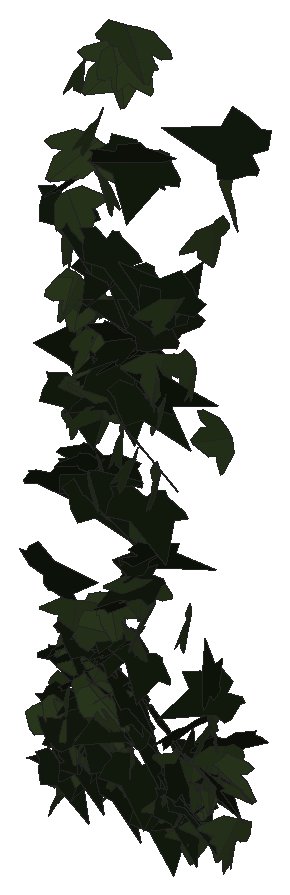
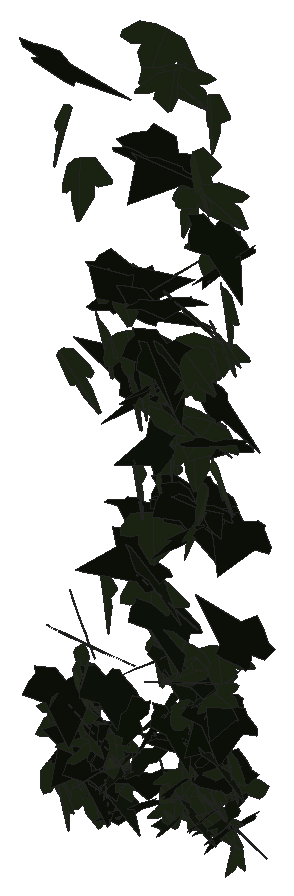
# SketchUp Ruby script. Lengths in inches.
U = 1.inch
M = Sketchup.active_model
def pt(a) = Geom::Point3d.new(a.map { |v| v * U })
def face(e, loops, mat)
  f = e.add_face(loops[0].map { |a| pt(a) })
  loops[1..].each { |l| e.add_face(l.map { |a| pt(a) }).erase! }
  f.material = f.back_material = mat if mat
  f
end
# faces: each face lists its corners as indices into pts; further lists are holes
def faces(e, pts, list, mat = nil) = list.each { |f| face(e, (f[0].is_a?(Array) ? f : [f]).map { |l| l.map { |i| pts[i] } }, mat) }
# xy, xz, yz: faces in a plane at the given z, y or x. An outline is a flat list of corners, or four numbers for a rectangle; further outlines are holes
def ring(l) = l.size == 4 ? [[l[0], l[1]], [l[2], l[1]], [l[2], l[3]], [l[0], l[3]]] : l.each_slice(2).to_a
def flat(e, list, mat, &to3) = list.each { |f| face(e, (f[0].is_a?(Array) ? f : [f]).map { |l| ring(l).map { |u, v| to3.(u, v) } }, mat) }
def xy(e, z, list, mat = nil) = flat(e, list, mat) { |x, y| [x, y, z] }
def xz(e, y, list, mat = nil) = flat(e, list, mat) { |x, z| [x, y, z] }
def yz(e, x, list, mat = nil) = flat(e, list, mat) { |y, z| [x, y, z] }
def lines(e, pts, list) = list.each { |a, b| e.add_line(pt(pts[a]), pt(pts[b])) }
# prism: a flat outline (further loops are holes) pulled along v
def prism(e, loops, v, mat = nil)
  f = face(e, loops, mat); d = Geom::Vector3d.new(v.map { |x| x * U })
  f.pushpull(f.normal.samedirection?(d) ? d.length : -d.length)
end
def box(e, o, s, mat = nil) = prism(e, [[o, [o[0] + s[0], o[1], o[2]], [o[0] + s[0], o[1] + s[1], o[2]], [o[0], o[1] + s[1], o[2]]]], [0, 0, s[2]], mat)
def at(x, y, z, deg = 0) = Geom::Transformation.translation(pt([x, y, z])) * Geom::Transformation.rotation(ORIGIN, Z_AXIS, deg.degrees)
def axes(o, x, y, z) = Geom::Transformation.new([*x, 0, *y, 0, *z, 0, *pt(o).to_a, 1])
def part(name) = M.definitions.add(name)
# library, detail: a bought-in or finely detailed component or shape, given as its bounding box
def library(name, o, s) = part(name).tap { |d| box(d.entities, o, s) }
def detail(e, o, s) = box(e.add_group.entities, o, s)
def put(e, d, t, mat = nil) = e.add_instance(d, t).tap { |i| i.material = mat if mat }
def group(e, t, mat = nil) = e.add_group.tap { |g| g.transformation = t; g.material = mat if mat }.entities
root = M.entities
M.materials.add("1026 AP 7946 SUNNY SIDE UP").color = [254, 231, 186]
M.materials.add("efeu1").color = [18, 25, 13]
M.materials.add("efeu2").color = [43, 57, 29]
c1 = part("ivyleaf_10")
p = [[0,0.5,-0.03],[-0.0625,2.02,-0.43],[-0.19,2.01,-0.46],[-0.54,1.05,-0.29],[-0.52,0.625,-0.18],[-0.83,0.76,-0.28],
  [-1.16,0.64,-0.33],[-1.15,0.33,-0.24],[-0.77,-0.39,0.02],[-0.3,-0.51,0.16],[0.04,-0.48,0.23],[-0.02,2.01,-0.4375],
  [-0.06,2.01,-0.43],[0.04,-0.49,0.23],[0.67,-0.49,0.14],[1.38,0.36,-0.2],[1.375,0.51,-0.24],[0.81,0.65,-0.19],
  [0.62,0.59,-0.15],[0.6,1.09,-0.28],[0.5,1.23,-0.31]]
faces(c1.entities,p,[[0,1,2,3,4,5,6,7,8,9,10],[11,12,0,13,14,15,16,17,18,19,20]],"efeu2")
c2 = part("ivyleaf_9")
p = [[1.54,2.16,1.25],[1.36,2.04,1.19],[-0.21,0.99,0.68],[-0.71,1.11,0.82],[-0.85,0.86,0.67],[-0.8,0.17,0.21],
  [-0.9,-0.01,0.1],[-0.67,-0.16,-0.02],[-0.08,-0.08,-0.05],[-0.03,-0.6,-0.4],[0.65,-0.88,-0.66],[0.83,-0.6,-0.49],
  [1.29,-0.42,-0.43],[1.8125,-0.07,-0.26],[1.21,0.44,0.15]]
faces(c2.entities,p,[[0,1,2,3,4,5,6,7,8,9,10,11,12,13,14]],"efeu1")
put(root,c1,axes([99.48,212.96,273.32],[-0.02906,0.13173,0.21889],[-0.30626,0.12835,-0.1038],[-0.27324,-0.15787,0.09306]),"1026 AP 7946 SUNNY SIDE UP")
put(root,c1,axes([99.28,212.93,269.21],[0.26104,-0.20482,-0.03217],[0.01718,0.04715,-0.26851],[0.32505,0.16199,0.04003]),"1026 AP 7946 SUNNY SIDE UP")
put(root,c1,axes([99.33,212.97,275.96],[0.25724,-0.22713,-0.0943],[-0.00591,0.10625,-0.28187],[0.38425,0.15368,0.05879]),"1026 AP 7946 SUNNY SIDE UP")
put(root,c2,axes([99.04,212.875,270.85],[0.02843,-0.03643,0.27976],[0.29208,-0.19871,-0.04134],[0.31714,0.18627,0.01299]),"1026 AP 7946 SUNNY SIDE UP")
put(root,c2,axes([99.59,212.82,268.3],[-0.23447,0.14999,0.07578],[-0.104,0.03674,-0.21682],[-0.26012,-0.14989,0.01838]),"1026 AP 7946 SUNNY SIDE UP")
put(root,c2,axes([99.51,212.96,276.91],[-0.07158,0.29227,-0.0364],[0.00245,-0.03719,-0.30491],[-0.46322,-0.04536,0.00402]),"1026 AP 7946 SUNNY SIDE UP")
put(root,c1,axes([99.38,212.6875,267.79],[-0.00639,-0.10073,-0.20656],[0.01108,0.19151,-0.10524],[0.36733,-0.00753,-0.00042]),"1026 AP 7946 SUNNY SIDE UP")
put(root,c2,axes([99.32,212.67,272.54],[0.26615,0.18266,-0.01135],[0.00617,-0.02019,-0.25743],[-0.3108,0.15602,-0.01483]),"1026 AP 7946 SUNNY SIDE UP")
put(root,c1,axes([99.16,212.77,268.875],[0.2529,0.11365,0.14396],[0.19708,0.06644,-0.19909],[-0.22215,0.18833,-0.01273]),"1026 AP 7946 SUNNY SIDE UP")
put(root,c1,axes([99.27,212.875,269.01],[0.14805,0.1932,0.05915],[0.04785,0.0451,-0.22619],[-0.33658,0.09139,-0.00614]),"1026 AP 7946 SUNNY SIDE UP")
put(root,c1,axes([99.42,213.03,270.15],[0.13651,0.14455,-0.1499],[-0.10188,-0.12882,-0.17869],[-0.32841,0.10005,-0.00687]),"1026 AP 7946 SUNNY SIDE UP")
put(root,c2,axes([99.72,212.87,274.45],[-0.04379,-0.02297,-0.29501],[-0.44997,-0.02165,0.03035],[-0.03748,0.28677,-0.01964]),"1026 AP 7946 SUNNY SIDE UP")
put(root,c2,axes([99.23,212.9,268.5],[0.24861,-0.20292,-0.05814],[-0.03895,0.05072,-0.26445],[0.3284,0.15963,0.01265]),"1026 AP 7946 SUNNY SIDE UP")
put(root,c2,axes([99.62,212.87,269.22],[-0.11625,0.20118,0.06581],[-0.06571,0.0487,-0.2258],[-0.3497,-0.07603,0.02055]),"1026 AP 7946 SUNNY SIDE UP")
put(root,c2,axes([99.44,212.87,269.83],[0.24397,0.14977,-0.08389],[-0.06946,-0.0716,-0.22232],[-0.28,0.14826,-0.01795]),"1026 AP 7946 SUNNY SIDE UP")
put(root,c2,axes([99.3,212.84,268.1875],[0.08772,-0.24399,-0.0776],[-0.01717,0.07334,-0.25735],[0.40052,0.05658,0.00596]),"1026 AP 7946 SUNNY SIDE UP")
put(root,c2,axes([99.48,212.79,270.02],[0.10433,0.20292,0.08704],[0.05126,0.07299,-0.22584],[-0.36587,0.06809,-0.00682]),"1026 AP 7946 SUNNY SIDE UP")
put(root,c1,axes([99.47,212.91,275.3],[0.29987,-0.17743,0.03416],[0.0212,-0.03575,-0.26798],[0.30601,0.17634,-0.01491]),"1026 AP 7946 SUNNY SIDE UP")
put(root,c2,axes([99.33,212.95,276.48],[0.05518,-0.29071,-0.04839],[-0.0112,0.04479,-0.3014],[0.46251,0.03577,-0.00152]),"1026 AP 7946 SUNNY SIDE UP")
put(root,c1,axes([99.58,212.82,270.58],[-0.27514,-0.15876,0.01353],[-0.00008,-0.02093,-0.24267],[0.27066,-0.1614,0.01368]),"1026 AP 7946 SUNNY SIDE UP")
put(root,c1,axes([99.64,212.89,268.63],[0.18742,-0.13295,-0.14177],[-0.13748,0.10261,-0.18356],[0.28505,0.1369,0.00468]),"1026 AP 7946 SUNNY SIDE UP")
put(root,c1,axes([99.63,212.93,268.2],[0.30089,0.03433,-0.12362],[-0.18268,-0.04895,-0.19237],[-0.09353,0.20606,-0.02198]),"1026 AP 7946 SUNNY SIDE UP")
put(root,c2,axes([99.29,212.95,268.93],[-0.01066,-0.02643,0.23627],[0.37545,-0.02589,0.00305],[0.04298,0.21961,0.03195]),"1026 AP 7946 SUNNY SIDE UP")
put(root,c1,axes([99.68,212.95,277.375],[0.37547,0.07924,-0.1682],[-0.22868,-0.07909,-0.25841],[-0.17176,0.27851,-0.02364]),"1026 AP 7946 SUNNY SIDE UP")
put(root,c1,axes([99.55,212.87,268.75],[0.11961,0.20132,-0.04717],[-0.02057,-0.04521,-0.22895],[-0.35022,0.07141,-0.00266]),"1026 AP 7946 SUNNY SIDE UP")
put(root,c1,axes([99.63,212.86,278.625],[0.04202,-0.24833,-0.11165],[0.01989,0.10238,-0.26486],[0.45467,0.01847,0.0219]),"1026 AP 7946 SUNNY SIDE UP")
put(root,c1,axes([99.54,212.95,275.21],[0.41653,0.05757,-0.00079],[0.00664,-0.02316,-0.26898],[-0.09753,0.24428,-0.02169]),"1026 AP 7946 SUNNY SIDE UP")
put(root,c1,axes([99.6,212.73,276.64],[0.13605,0.27126,0.08601],[-0.0259,0.09035,-0.28967],[-0.44482,0.0777,0.04317]),"1026 AP 7946 SUNNY SIDE UP")
put(root,c2,axes([99.6,212.8,269.52],[0.15571,0.15469,0.14055],[0.10084,0.11497,-0.19082],[-0.32701,0.10911,0.00808]),"1026 AP 7946 SUNNY SIDE UP")
put(root,c1,axes([99.71,213.16,274.98],[-0.06034,-0.2179,0.12437],[-0.01126,-0.11935,-0.23773],[0.42132,-0.0344,0.01146]),"1026 AP 7946 SUNNY SIDE UP")
put(root,c2,axes([99.64,212.72,268.61],[-0.29105,-0.01711,0.1575],[0.24634,0.02724,0.18456],[-0.05209,0.22442,-0.0072]),"1026 AP 7946 SUNNY SIDE UP")
put(root,c2,axes([99.54,212.95,273.78],[-0.14208,-0.21245,-0.09578],[0.11469,0.06538,-0.24043],[0.37225,-0.10123,0.03752]),"1026 AP 7946 SUNNY SIDE UP")
put(root,c2,axes([99.58,212.84,269.98],[0.20095,-0.1581,-0.11715],[-0.13095,0.07602,-0.20984],[0.29682,0.14058,-0.01326]),"1026 AP 7946 SUNNY SIDE UP")
put(root,c2,axes([99.54,212.93,268.38],[0.09931,-0.25091,-0.03775],[-0.0209,0.03296,-0.26631],[0.39785,0.06436,-0.00457]),"1026 AP 7946 SUNNY SIDE UP")
put(root,c1,axes([99.71,212.98,272.96],[-0.22119,0.20081,0.0047],[-0.02725,-0.00831,-0.25567],[-0.33981,-0.13005,0.01745]),"1026 AP 7946 SUNNY SIDE UP")
put(root,c2,axes([99.5,212.91,270.19],[0.21501,-0.21942,-0.0849],[-0.00202,0.09331,-0.26154],[0.36786,0.12876,0.04819]),"1026 AP 7946 SUNNY SIDE UP")
put(root,c1,axes([99.78,212.96,277.76],[0.06086,-0.29776,-0.03273],[-0.00454,0.02996,-0.30915],[0.47056,0.0388,0.00125]),"1026 AP 7946 SUNNY SIDE UP")
put(root,c1,axes([99.7,212.92,273.89],[-0.33973,-0.11641,-0.08991],[0.1576,0.0016,-0.2436],[0.18388,-0.21645,0.04266]),"1026 AP 7946 SUNNY SIDE UP")
put(root,c1,axes([99.78,212.91,268.77],[0.04086,-0.20317,0.08096],[0.02729,-0.07687,-0.22],[0.36859,0.02822,0.00732]),"1026 AP 7946 SUNNY SIDE UP")
put(root,c2,axes([99.82,213.0625,268.29],[-0.26926,0.02251,-0.14891],[0.19446,-0.10204,-0.15862],[-0.14011,-0.18487,0.06602]),"1026 AP 7946 SUNNY SIDE UP")
put(root,c1,axes([99.9,212.85,268.57],[-0.34195,-0.06555,0.06616],[-0.08761,-0.04262,-0.22597],[0.12657,-0.20661,0.02233]),"1026 AP 7946 SUNNY SIDE UP")
put(root,c1,axes([99.9,212.89,269.72],[-0.28529,-0.17399,0.09757],[-0.0401,-0.10814,-0.25299],[0.30965,-0.1743,0.05714]),"1026 AP 7946 SUNNY SIDE UP")
put(root,c1,axes([99.84,212.91,274.57],[0.17858,0.17914,-0.14354],[-0.12692,-0.11423,-0.22393],[-0.36054,0.12894,0.00774]),"1026 AP 7946 SUNNY SIDE UP")
put(root,c2,axes([99.93,212.87,272.83],[0.14729,0.21051,-0.17033],[-0.08716,-0.15741,-0.23803],[-0.41296,0.10831,-0.01051]),"1026 AP 7946 SUNNY SIDE UP")
put(root,c2,axes([99.99,212.87,272.92],[0.21407,0.1349,-0.21574],[-0.1958,-0.17084,-0.19705],[-0.34042,0.1831,-0.02233]),"1026 AP 7946 SUNNY SIDE UP")
put(root,c1,axes([99.84,212.89,272.5],[-0.11595,0.271,0.03562],[-0.01419,0.03178,-0.28915],[-0.42904,-0.07429,-0.00006]),"1026 AP 7946 SUNNY SIDE UP")
put(root,c1,axes([99.93,212.88,273.59],[-0.13026,-0.27077,-0.03588],[0.02259,0.03041,-0.29149],[0.42837,-0.08394,0.00446]),"1026 AP 7946 SUNNY SIDE UP")
put(root,c2,axes([99.91,213.12,275.68],[-0.3555,-0.03039,-0.15172],[0.24116,-0.08919,-0.2061],[-0.04528,-0.23638,0.09345]),"1026 AP 7946 SUNNY SIDE UP")
put(root,c1,axes([99.76,212.85,270.33],[-0.04557,-0.09391,-0.22584],[0.26716,0.14635,-0.08967],[0.28424,-0.15261,0.04808]),"1026 AP 7946 SUNNY SIDE UP")
put(root,c2,axes([99.67,212.9375,269.35],[0.32432,-0.07494,0.09486],[0.12733,-0.05292,-0.21939],[0.15197,0.20427,-0.01861]),"1026 AP 7946 SUNNY SIDE UP")
put(root,c1,axes([99.91,212.8,269.12],[-0.31655,0.0954,-0.0812],[0.10269,-0.0505,-0.22427],[-0.18113,-0.19536,0.01476]),"1026 AP 7946 SUNNY SIDE UP")
put(root,c2,axes([100.16,212.93,270.15],[-0.22318,0.1661,-0.06961],[0.02126,-0.07461,-0.22475],[-0.30341,-0.12741,0.03546]),"1026 AP 7946 SUNNY SIDE UP")
put(root,c2,axes([99.79,212.88,272.4],[0.12537,-0.21985,-0.16406],[0.01995,0.16756,-0.23262],[0.42524,0.05695,0.05928]),"1026 AP 7946 SUNNY SIDE UP")
put(root,c1,axes([100.07,212.77,277.13],[-0.29153,0.18982,0.05644],[-0.0697,0.03056,-0.27342],[-0.32596,-0.17631,0.00799]),"1026 AP 7946 SUNNY SIDE UP")
put(root,c1,axes([100,213.04,268.82],[0.15013,0.19121,-0.04039],[-0.02115,-0.03854,-0.22603],[-0.33102,0.08919,-0.00388]),"1026 AP 7946 SUNNY SIDE UP")
put(root,c2,axes([99.87,212.9,272.69],[-0.16585,-0.16563,-0.21064],[0.21774,0.15119,-0.1998],[0.35048,-0.17231,0.02445]),"1026 AP 7946 SUNNY SIDE UP")
put(root,c2,axes([99.99,213.18,270.21],[-0.21047,-0.18459,0.00949],[0.10301,-0.05343,-0.22284],[0.29656,-0.11245,0.08414]),"1026 AP 7946 SUNNY SIDE UP")
put(root,c2,axes([100.27,212.91,273.99],[-0.35524,0.11989,-0.03775],[-0.00129,-0.07284,-0.2503],[-0.2129,-0.19961,0.06451]),"1026 AP 7946 SUNNY SIDE UP")
put(root,c2,axes([100.18,212.97,269.51],[-0.01621,0.21772,0.01632],[-0.01153,0.01212,-0.23305],[-0.37002,-0.00991,0.00655]),"1026 AP 7946 SUNNY SIDE UP")
put(root,c1,axes([99.96,213.02,270.68],[0.35551,-0.00348,0.09238],[0.14556,-0.01948,-0.2238],[0.01806,0.22568,-0.01472]),"1026 AP 7946 SUNNY SIDE UP")
put(root,c1,axes([100.44,212.86,273.875],[0.03534,0.04698,0.29322],[-0.41166,-0.11595,0.04038],[0.18952,-0.26062,0.03302]),"1026 AP 7946 SUNNY SIDE UP")
put(root,c2,axes([100,212.9,268.65],[0.11642,-0.22462,-0.12154],[-0.04103,0.11417,-0.24277],[0.3959,0.07789,0.01058]),"1026 AP 7946 SUNNY SIDE UP")
put(root,c1,axes([99.98,212.76,269.43],[0.23136,0.12898,0.14159],[0.17872,0.07828,-0.19933],[-0.2552,0.17175,-0.01124]),"1026 AP 7946 SUNNY SIDE UP")
put(root,c1,axes([100.14,213.03,268.28],[0.14338,0.1858,-0.05314],[-0.02499,-0.05046,-0.21907],[-0.3266,0.08543,-0.00657]),"1026 AP 7946 SUNNY SIDE UP")
put(root,c1,axes([100.28,212.92,278.91],[0.40825,0.05973,-0.15606],[-0.21615,-0.07359,-0.27244],[-0.13817,0.29162,-0.0349]),"1026 AP 7946 SUNNY SIDE UP")
put(root,c2,axes([100.4,212.85,270.35],[-0.23754,0.18054,-0.10144],[0.00838,-0.11457,-0.23726],[-0.34789,-0.12603,0.06355]),"1026 AP 7946 SUNNY SIDE UP")
put(root,c2,axes([100.41,212.96,269.15],[-0.3875,-0.05497,0.05522],[-0.06866,-0.05214,-0.24838],[0.10897,-0.22831,0.03988]),"1026 AP 7946 SUNNY SIDE UP")
put(root,c2,axes([100.42,212.86,274.82],[-0.35603,0.13221,-0.10197],[0.08201,-0.10063,-0.26014],[-0.26597,-0.208,0.05629]),"1026 AP 7946 SUNNY SIDE UP")
put(root,c2,axes([100.04,212.92,276.12],[0.09562,-0.28949,-0.02436],[0.02882,0.02626,-0.30364],[0.4556,0.0591,0.02432]),"1026 AP 7946 SUNNY SIDE UP")
put(root,c1,axes([100.28,212.96,268.35],[0.02651,-0.18688,0.13091],[0.01109,-0.12459,-0.20247],[0.38123,0.01662,-0.00322]),"1026 AP 7946 SUNNY SIDE UP")
put(root,c2,axes([100.1,212.9375,268.13],[0.14393,-0.24195,0.01973],[0.00408,-0.02096,-0.26657],[0.38178,0.09144,-0.00459]),"1026 AP 7946 SUNNY SIDE UP")
put(root,c2,axes([100.37,212.88,274.87],[0.29758,0.11706,-0.17039],[-0.24601,-0.07141,-0.22595],[-0.23102,0.22683,0.02113]),"1026 AP 7946 SUNNY SIDE UP")
put(root,c1,axes([100.22,212.95,278.91],[0.17131,0.28486,-0.03155],[-0.012,-0.03159,-0.31435],[-0.45062,0.10913,-0.00362]),"1026 AP 7946 SUNNY SIDE UP")
put(root,c2,axes([100.24,213.16,275.69],[-0.20341,-0.22214,-0.0267],[0.06632,0.00376,-0.26791],[0.3731,-0.12178,0.03307]),"1026 AP 7946 SUNNY SIDE UP")
put(root,c2,axes([100.44,212.84,270.96],[0.06915,0.24636,-0.03721],[-0.06913,-0.03138,-0.26518],[-0.41746,0.04601,0.03775]),"1026 AP 7946 SUNNY SIDE UP")
put(root,c2,axes([100.45,212.82,274.625],[-0.01772,0.26378,0.00074],[0.00386,-0.00266,-0.28264],[-0.44778,-0.01046,-0.00247]),"1026 AP 7946 SUNNY SIDE UP")
put(root,c1,axes([100.32,212.81,273.36],[0.12602,-0.26048,-0.08412],[0.03929,0.09024,-0.27577],[0.42673,0.06861,0.05023]),"1026 AP 7946 SUNNY SIDE UP")
put(root,c1,axes([100.39,212.9,270.42],[-0.3177,0.1625,0.01073],[-0.05377,-0.02458,-0.26234],[-0.2709,-0.1857,0.03948]),"1026 AP 7946 SUNNY SIDE UP")
put(root,c2,axes([100.27,212.875,269.67],[0.2186,-0.18155,-0.08384],[-0.07996,0.05968,-0.23743],[0.32436,0.13707,-0.00203]),"1026 AP 7946 SUNNY SIDE UP")
put(root,c1,axes([100.46,212.85,273.02],[0.04737,-0.25588,-0.02137],[0.00548,0.01707,-0.27528],[0.43526,0.02763,0.00579]),"1026 AP 7946 SUNNY SIDE UP")
put(root,c1,axes([100.32,212.93,268.55],[0.22452,-0.11139,0.15662],[0.17906,-0.10382,-0.18634],[0.25807,0.16895,-0.00697]),"1026 AP 7946 SUNNY SIDE UP")
put(root,c2,axes([100.36,212.89,274.27],[-0.12896,-0.26618,-0.08498],[0.03395,0.07808,-0.28647],[0.43616,-0.08478,-0.00283]),"1026 AP 7946 SUNNY SIDE UP")
put(root,c2,axes([100.68,212.93,271.59],[-0.16074,0.22316,0.07734],[-0.05496,0.06156,-0.2586],[-0.39286,-0.09992,0.00453]),"1026 AP 7946 SUNNY SIDE UP")
put(root,c2,axes([100.36,212.95,269.45],[0.14665,-0.1915,-0.13252],[-0.11295,0.10266,-0.22283],[0.36785,0.10787,-0.01559]),"1026 AP 7946 SUNNY SIDE UP")
put(root,c1,axes([100.46,212.89,279.35],[-0.47575,-0.00317,-0.05935],[0.08962,-0.06362,-0.30524],[-0.01392,-0.30135,0.06322]),"1026 AP 7946 SUNNY SIDE UP")
put(root,c2,axes([100.35,212.74,277.63],[0.37772,0.16921,0.0273],[0.0626,-0.01024,-0.29764],[-0.28312,0.22349,-0.02939]),"1026 AP 7946 SUNNY SIDE UP")
put(root,c2,axes([100.6875,212.97,271.36],[-0.39261,0.08166,-0.04319],[0.04835,-0.04275,-0.26116],[-0.14771,-0.23104,0.02932]),"1026 AP 7946 SUNNY SIDE UP")
put(root,c1,axes([100.5625,212.93,272.22],[-0.36271,-0.12942,0.00819],[0.00521,-0.02303,-0.26679],[0.2202,-0.21263,0.0198]),"1026 AP 7946 SUNNY SIDE UP")
put(root,c1,axes([100.62,212.91,271.21],[-0.32892,-0.14652,0.00674],[0.00875,-0.02037,-0.25953],[0.24897,-0.19286,0.01802]),"1026 AP 7946 SUNNY SIDE UP")
put(root,c2,axes([100.35,212.92,273.45],[0.34348,-0.16354,0.00621],[-0.00416,-0.01564,-0.27836],[0.27791,0.20189,-0.01184]),"1026 AP 7946 SUNNY SIDE UP")
put(root,c2,axes([100.59,212.95,277.57],[-0.35898,-0.16058,-0.11979],[0.21814,-0.00453,-0.27635],[0.22152,-0.25575,0.07802]),"1026 AP 7946 SUNNY SIDE UP")
put(root,c2,axes([101.07,212.85,275.26],[-0.26822,0.0676,0.23898],[-0.36265,0.03755,-0.18607],[-0.11134,-0.28517,0.03036]),"1026 AP 7946 SUNNY SIDE UP")
put(root,c2,axes([100.61,212.9,268.51],[-0.16539,-0.22609,-0.07074],[0.06131,0.05611,-0.2563],[0.36586,-0.11161,0.01097]),"1026 AP 7946 SUNNY SIDE UP")
put(root,c2,axes([100.62,212.95,270.16],[-0.10872,-0.21317,0.08222],[0.01239,-0.08455,-0.23737],[0.38606,-0.05732,0.03077]),"1026 AP 7946 SUNNY SIDE UP")
put(root,c2,axes([100.52,213.08,268.79],[0.03728,-0.19834,0.12239],[0.05234,-0.11384,-0.21457],[0.38731,0.03448,0.01722]),"1026 AP 7946 SUNNY SIDE UP")
put(root,c1,axes([100.72,212.86,270.85],[0.16693,-0.24972,0.04839],[0.00635,-0.05077,-0.27935],[0.39991,0.10504,-0.01576]),"1026 AP 7946 SUNNY SIDE UP")
put(root,c1,axes([100.77,212.89,274.38],[0.26544,-0.21719,-0.09756],[-0.00909,0.11102,-0.27587],[0.37168,0.15783,0.06293]),"1026 AP 7946 SUNNY SIDE UP")
put(root,c2,axes([100.55,212.88,274.14],[0.1415,-0.22232,-0.16982],[0.01749,0.17483,-0.23746],[0.43365,0.06549,0.06499]),"1026 AP 7946 SUNNY SIDE UP")
put(root,c2,axes([100.65,212.94,272.49],[-0.14992,-0.20795,-0.11923],[0.16831,0.07215,-0.23309],[0.36098,-0.12001,0.05916]),"1026 AP 7946 SUNNY SIDE UP")
put(root,c2,axes([101.14,212.87,275.52],[-0.01803,0.03838,0.30287],[-0.4315,0.10944,-0.02512],[-0.17559,-0.27287,0.03064]),"1026 AP 7946 SUNNY SIDE UP")
put(root,c1,axes([100.85,212.89,272.875],[0.16096,-0.2538,-0.07901],[-0.00153,0.08033,-0.27997],[0.41624,0.09844,0.02952]),"1026 AP 7946 SUNNY SIDE UP")
put(root,c2,axes([100.6,212.91,271.66],[0.29481,0.08255,0.17705],[0.2569,0.0642,-0.20488],[-0.17729,0.23029,-0.00247]),"1026 AP 7946 SUNNY SIDE UP")
put(root,c1,axes([100.99,212.86,274.69],[-0.24207,-0.24465,0.04507],[0.01156,-0.05753,-0.29575],[0.39102,-0.14976,0.03664]),"1026 AP 7946 SUNNY SIDE UP")
put(root,c1,axes([100.94,212.875,274.125],[0.24126,-0.24372,-0.03744],[0.00989,0.04506,-0.29491],[0.38703,0.15078,0.03088]),"1026 AP 7946 SUNNY SIDE UP")
put(root,c2,axes([100.73,213.03,269.3125],[0.24082,-0.17664,0.04312],[0.01912,-0.04537,-0.2423],[0.30785,0.141,-0.01869]),"1026 AP 7946 SUNNY SIDE UP")
put(root,c2,axes([100.64,212.875,274.27],[0.1699,-0.03429,0.27561],[0.35017,-0.15162,-0.11349],[0.23981,0.2457,-0.02955]),"1026 AP 7946 SUNNY SIDE UP")
put(root,c2,axes([100.94,212.96,267.92],[-0.05836,-0.25387,-0.02134],[0.03541,0.01613,-0.26342],[0.39876,-0.03859,0.02027]),"1026 AP 7946 SUNNY SIDE UP")
put(root,c1,axes([101.16,212.86,275.57],[-0.18384,-0.27144,0.03032],[-0.00192,-0.03317,-0.30442],[0.42958,-0.11632,0.01161]),"1026 AP 7946 SUNNY SIDE UP")
put(root,c2,axes([101.05,212.87,275.34],[-0.18638,-0.04749,0.27455],[0.34742,0.15161,0.12983],[-0.24663,0.24946,-0.02459]),"1026 AP 7946 SUNNY SIDE UP")
put(root,c2,axes([101.37,212.8,268.1],[-0.06862,0.23708,0.09503],[-0.12432,0.07496,-0.24007],[-0.37939,-0.06744,0.06148]),"1026 AP 7946 SUNNY SIDE UP")
put(root,c1,axes([101.2,212.75,268.37],[0.12755,-0.09339,0.24456],[-0.14189,0.22308,0.12321],[-0.37602,-0.11586,0.03647]),"1026 AP 7946 SUNNY SIDE UP")
put(root,c1,axes([101.22,212.875,268.22],[-0.20229,-0.22343,0.01479],[0.03411,-0.03036,-0.26348],[0.35053,-0.12599,0.03417]),"1026 AP 7946 SUNNY SIDE UP")
put(root,c1,axes([101.3,212.95,268.22],[0.10279,-0.2372,-0.08759],[0.00136,0.08667,-0.2519],[0.3955,0.06135,0.02363]),"1026 AP 7946 SUNNY SIDE UP")
put(root,c2,axes([101.4,212.95,268.44],[0.08378,0.24974,-0.05161],[-0.00903,-0.05144,-0.26332],[-0.40086,0.05335,-0.00486]),"1026 AP 7946 SUNNY SIDE UP")
put(root,c1,axes([101.43,212.83,268.81],[-0.40336,-0.00395,0.06198],[-0.09352,-0.02733,-0.26313],[0.01583,-0.26207,0.02496]),"1026 AP 7946 SUNNY SIDE UP")
put(root,c1,axes([101.37,212.8,268.09],[-0.15995,0.22579,0.07449],[-0.09987,0.04843,-0.25204],[-0.35853,-0.11422,0.03698]),"1026 AP 7946 SUNNY SIDE UP")
put(root,c1,axes([101.37,212.9375,268.83],[-0.33288,0.15141,0.02559],[-0.05124,-0.00451,-0.26715],[-0.23554,-0.213,0.02196]),"1026 AP 7946 SUNNY SIDE UP")
put(root,c2,axes([101.125,212.91,268.44],[0.25845,-0.20391,-0.01206],[0.00452,0.01586,-0.26943],[0.32103,0.16394,0.01351]),"1026 AP 7946 SUNNY SIDE UP")
put(root,c2,axes([101.5,212.7,269.51],[-0.03593,0.26633,-0.04534],[-0.00192,-0.04579,-0.27559],[-0.42484,-0.02232,0.00508]),"1026 AP 7946 SUNNY SIDE UP")
put(root,c2,axes([101.63,212.93,268.87],[-0.11608,0.17153,0.19232],[-0.15749,0.15779,-0.19024],[-0.36499,-0.12264,0.02092]),"1026 AP 7946 SUNNY SIDE UP")
put(root,c1,axes([101.39,212.87,270.98],[0.12108,-0.25815,-0.06323],[0.02057,0.06602,-0.27533],[0.41619,0.07184,0.032]),"1026 AP 7946 SUNNY SIDE UP")
put(root,c2,axes([101.25,212.9,268.2],[0.02881,-0.25957,-0.00555],[0.00717,0.00424,-0.26801],[0.40814,0.01825,0.0051]),"1026 AP 7946 SUNNY SIDE UP")
put(root,c2,axes([101.4375,212.71,268.55],[-0.10847,-0.09287,0.25172],[0.19122,0.2129,0.11973],[-0.3647,0.13925,-0.01209]),"1026 AP 7946 SUNNY SIDE UP")
put(root,c1,axes([101.42,212.88,274.73],[0.27423,-0.2312,-0.04249],[0.00149,0.05045,-0.29636],[0.36893,0.17166,0.03278]),"1026 AP 7946 SUNNY SIDE UP")
put(root,c2,axes([101.32,212.98,268.37],[0.08621,-0.25016,-0.03623],[0.01981,0.0372,-0.2628],[0.39642,0.05255,0.02101]),"1026 AP 7946 SUNNY SIDE UP")
put(root,c1,axes([101.61,212.875,267.95],[-0.18234,-0.227,0.04141],[0.0069,-0.04859,-0.26155],[0.36278,-0.11317,0.02579]),"1026 AP 7946 SUNNY SIDE UP")
put(root,c1,axes([101.46,212.96,268.64],[0.30442,0.17131,0.03509],[0.04706,0.01609,-0.2661],[-0.27028,0.19575,-0.00681]),"1026 AP 7946 SUNNY SIDE UP")
put(root,c1,axes([101.55,212.95,268.55],[0.02499,0.25244,0.06924],[-0.0554,0.06738,-0.25721],[-0.40644,0.00634,0.03932]),"1026 AP 7946 SUNNY SIDE UP")
put(root,c2,axes([101.56,212.93,268.68],[0.38423,0.08772,-0.02647],[-0.03386,-0.01748,-0.2674],[-0.13991,0.24513,-0.00797]),"1026 AP 7946 SUNNY SIDE UP")
put(root,c2,axes([101.47,212.93,268.78],[0.38887,-0.08309,0.00369],[-0.00924,-0.03013,-0.26711],[0.13048,0.2455,-0.02991]),"1026 AP 7946 SUNNY SIDE UP")
put(root,c1,axes([101.58,213.01,268.77],[0.31551,-0.12065,0.11447],[0.16305,-0.04411,-0.24102],[0.20077,0.22542,0.01585]),"1026 AP 7946 SUNNY SIDE UP")
put(root,c1,axes([101.76,212.9,269.52],[0.12498,-0.24234,0.08164],[0.01287,-0.08198,-0.26265],[0.40139,0.07809,-0.017]),"1026 AP 7946 SUNNY SIDE UP")
put(root,c1,axes([101.71,212.91,269.78],[-0.19611,0.22392,-0.06986],[0.02426,-0.07024,-0.26366],[-0.36767,-0.12407,0.01986]),"1026 AP 7946 SUNNY SIDE UP")
put(root,c2,axes([101.96,212.92,270.09],[-0.41927,0.0111,0.00961],[-0.01977,-0.09339,-0.25794],[-0.01124,-0.24992,0.09515]),"1026 AP 7946 SUNNY SIDE UP")
put(root,c2,axes([101.9,212.7,270.17],[0.00931,0.06041,0.27656],[-0.03036,0.26761,-0.06011],[-0.43108,-0.01754,0.0102]),"1026 AP 7946 SUNNY SIDE UP")
put(root,c1,axes([101.79,212.85,276.92],[-0.09483,-0.28952,-0.06801],[0.05773,0.05789,-0.30335],[0.46277,-0.06655,0.02391]),"1026 AP 7946 SUNNY SIDE UP")
put(root,c1,axes([102.05,212.76,273.98],[0.23183,-0.13645,-0.23494],[-0.25113,0.16185,-0.20589],[0.33269,0.21725,0.0083]),"1026 AP 7946 SUNNY SIDE UP")
put(root,c1,axes([101.91,212.96,269.15],[-0.17189,-0.23867,0.01198],[0.03252,-0.02367,-0.26897],[0.37443,-0.10751,0.02886]),"1026 AP 7946 SUNNY SIDE UP")
put(root,c2,axes([101.99,212.9375,269.39],[0.13452,0.24231,-0.06828],[-0.0212,-0.06694,-0.26495],[-0.39502,0.08611,-0.00903]),"1026 AP 7946 SUNNY SIDE UP")
put(root,c1,axes([102.06,212.98,268.11],[-0.16427,-0.21631,0.09202],[-0.00069,-0.09895,-0.24461],[0.36872,-0.09656,0.04054]),"1026 AP 7946 SUNNY SIDE UP")
put(root,c1,axes([102,213,267.86],[0.23228,-0.20584,-0.03392],[0.01165,0.0441,-0.25873],[0.32729,0.14452,0.03328]),"1026 AP 7946 SUNNY SIDE UP")
put(root,c1,axes([101.85,212.9,268.97],[-0.28745,-0.10133,-0.16627],[0.2688,0.00992,-0.20657],[0.13068,-0.24328,0.05916]),"1026 AP 7946 SUNNY SIDE UP")
put(root,c1,axes([102.07,212.84,277.59],[-0.2203,0.2558,0.09569],[-0.09147,0.07224,-0.29961],[-0.41723,-0.1509,0.01516]),"1026 AP 7946 SUNNY SIDE UP")
put(root,c2,axes([102.44,212.82,278.33],[-0.30146,0.116,0.21988],[-0.31993,0.07035,-0.22796],[-0.20702,-0.27764,0.0321]),"1026 AP 7946 SUNNY SIDE UP")
